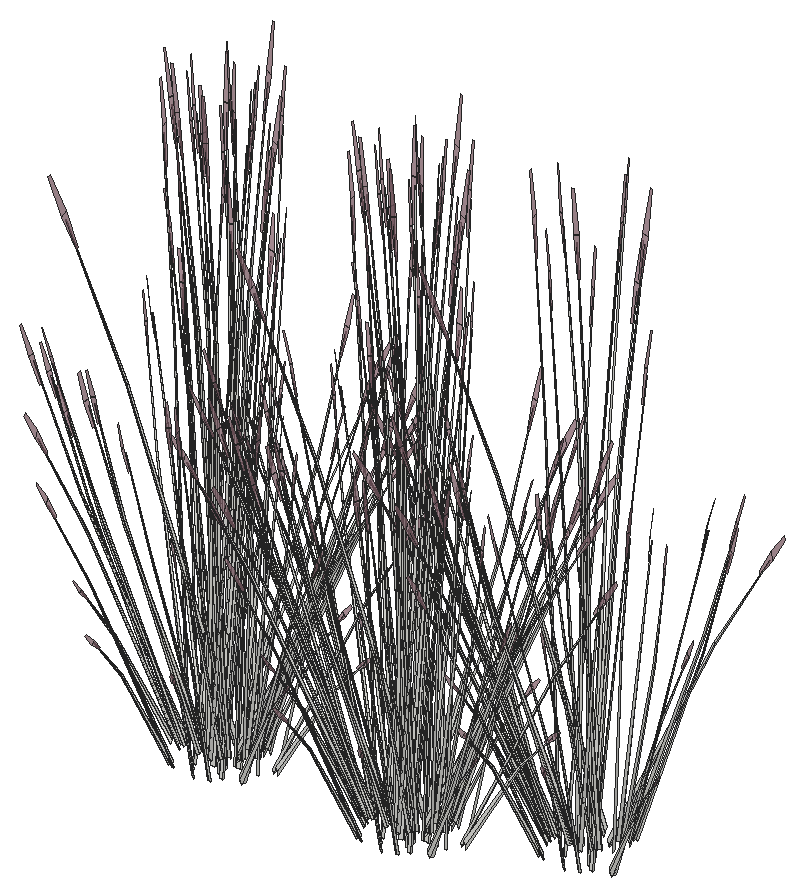
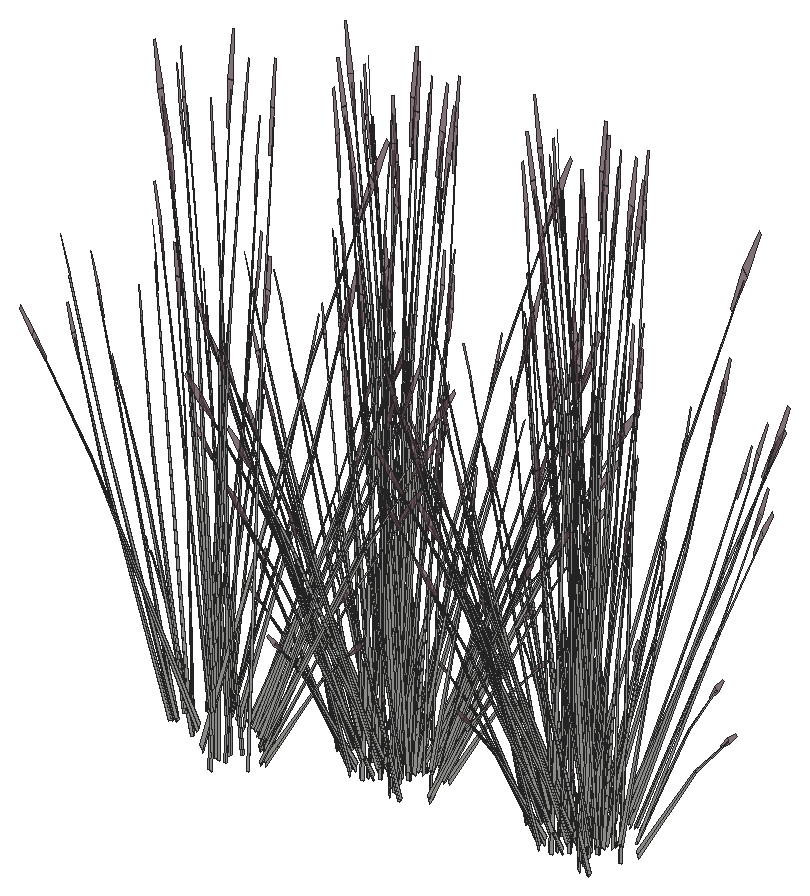
# SketchUp Ruby script. Lengths in inches.
U = 1.inch
M = Sketchup.active_model
def pt(a) = Geom::Point3d.new(a.map { |v| v * U })
def face(e, loops, mat)
  f = e.add_face(loops[0].map { |a| pt(a) })
  loops[1..].each { |l| e.add_face(l.map { |a| pt(a) }).erase! }
  f.material = f.back_material = mat if mat
  f
end
# faces: each face lists its corners as indices into pts; further lists are holes
def faces(e, pts, list, mat = nil) = list.each { |f| face(e, (f[0].is_a?(Array) ? f : [f]).map { |l| l.map { |i| pts[i] } }, mat) }
# xy, xz, yz: faces in a plane at the given z, y or x. An outline is a flat list of corners, or four numbers for a rectangle; further outlines are holes
def ring(l) = l.size == 4 ? [[l[0], l[1]], [l[2], l[1]], [l[2], l[3]], [l[0], l[3]]] : l.each_slice(2).to_a
def flat(e, list, mat, &to3) = list.each { |f| face(e, (f[0].is_a?(Array) ? f : [f]).map { |l| ring(l).map { |u, v| to3.(u, v) } }, mat) }
def xy(e, z, list, mat = nil) = flat(e, list, mat) { |x, y| [x, y, z] }
def xz(e, y, list, mat = nil) = flat(e, list, mat) { |x, z| [x, y, z] }
def yz(e, x, list, mat = nil) = flat(e, list, mat) { |y, z| [x, y, z] }
def lines(e, pts, list) = list.each { |a, b| e.add_line(pt(pts[a]), pt(pts[b])) }
# prism: a flat outline (further loops are holes) pulled along v
def prism(e, loops, v, mat = nil)
  f = face(e, loops, mat); d = Geom::Vector3d.new(v.map { |x| x * U })
  f.pushpull(f.normal.samedirection?(d) ? d.length : -d.length)
end
def box(e, o, s, mat = nil) = prism(e, [[o, [o[0] + s[0], o[1], o[2]], [o[0] + s[0], o[1] + s[1], o[2]], [o[0], o[1] + s[1], o[2]]]], [0, 0, s[2]], mat)
def at(x, y, z, deg = 0) = Geom::Transformation.translation(pt([x, y, z])) * Geom::Transformation.rotation(ORIGIN, Z_AXIS, deg.degrees)
def axes(o, x, y, z) = Geom::Transformation.new([*x, 0, *y, 0, *z, 0, *pt(o).to_a, 1])
def part(name) = M.definitions.add(name)
# library, detail: a bought-in or finely detailed component or shape, given as its bounding box
def library(name, o, s) = part(name).tap { |d| box(d.entities, o, s) }
def detail(e, o, s) = box(e.add_group.entities, o, s)
def put(e, d, t, mat = nil) = e.add_instance(d, t).tap { |i| i.material = mat if mat }
def group(e, t, mat = nil) = e.add_group.tap { |g| g.transformation = t; g.material = mat if mat }.entities
root = M.entities
M.materials.add("LightPink_Translucent").color = [144, 107, 117]
M.materials["LightPink_Translucent"].alpha = 0.75
c1 = part("blade")
p = [[2.15,0.21,22],[0,0.17,0],[0.09,0.45,0],[2.18,0.31,22],[2.29,0.31,22],[0.38,0.45,0],
  [2.48,0.24,33],[2.49,0.24,33],[2.48,0.22,33]]
faces(c1.entities,p,[[0,1,2,3],[4,5,2,3],[6,3,4,7],[8,0,3,6]])
c2 = part("seeds")
p = [[0.3,-0.1,1.38],[-0.01,-0.03,1.59],[-0.01,-0.03,0.03],[0.14,-0.07,-0.07],[0.29,-0.03,3],[0.15,0.01,3.11]]
faces(c2.entities,p,[[0,1,2,3],[1,0,4,5]],"LightPink_Translucent")
c3 = part("blade with seeds")
put(c3.entities,c1,at(0,0,0))
put(c3.entities,c2,axes([2.4,0.25,30.99],[1.5799,-0.05474,1.17369],[-0.12525,1.92788,0.29478],[-0.07173,-0.02425,1.56792]))
put(root,c3,axes([361.61,51.9,259.53],[-0.43232,-0.38257,-0.35414],[0.49364,-0.36215,0.4572],[-0.25081,-0.0551,0.87481]))
put(root,c3,axes([362.22,54.17,258.875],[0.18977,-0.18775,1.71376],[0.47917,0.50677,0.13857],[-0.32866,0.23079,0.73262]))
put(root,c3,axes([361.08,54.67,259.53],[-0.66138,0.08733,-0.35414],[-0.17464,-0.49921,0.4572],[-0.18953,0.13408,0.87481]))
put(root,c3,axes([360.57,52.82,257.77],[0.48508,-0.04372,1.1486],[-0.3077,0.38525,0.84392],[-0.23971,-0.05779,0.25299]))
put(root,c3,axes([362.08,54.64,258.875],[0.14147,-0.21002,1.71376],[0.59349,0.43464,0.13857],[-0.26773,0.27089,0.73262]))
put(root,c3,axes([361.625,54.72,259.68],[0.19519,0.55794,-0.51099],[-0.73919,0.0976,-0.3958],[-0.21183,0.14986,0.97773]))
put(root,c3,axes([363.39,51.43,259.98],[-0.64788,-0.29534,-0.71045],[0.46044,-0.51755,0.08574],[-0.23473,-0.17635,1.00501]))
put(root,c3,axes([363.09,51.44,259.68],[-0.74975,0.14525,-0.51099],[-0.13115,-0.55007,-0.3958],[-0.20138,-0.15763,0.97773]))
put(root,c3,axes([362.66,50.625,257.59],[-0.04601,0.19989,1.43002],[-0.67263,0.16733,-0.30754],[-0.15723,-0.25836,0.61141]))
put(root,c3,axes([362.88,51.14,258.875],[0.17368,0.19618,1.71376],[-0.80256,0.16516,0.13857],[-0.18139,-0.30799,0.73262]))
put(root,c3,axes([363.16,51.04,259.53],[-0.11735,-0.49217,-0.35414],[0.67083,-0.12996,0.4572],[-0.18018,-0.14104,0.87481]))
put(root,c3,axes([362.24,55.82,259.53],[-0.5141,0.32171,-0.35414],[-0.48666,-0.36734,0.4572],[-0.07405,0.18664,0.87481]))
put(root,c3,axes([364.9375,54.77,258.33],[0.65659,0.2464,1.51261],[-0.64324,0.53082,0.59816],[-0.28812,-0.31461,1.26806]))
put(root,c3,axes([362.43,50.3,257.77],[0.39634,0.21267,1.1486],[-0.57721,0.12784,0.84392],[-0.1235,-0.16344,0.25299]))
put(root,c3,axes([362.57,57.07,257.77],[-0.01966,-0.36332,1.1486],[0.49135,0.25914,0.84392],[-0.09663,0.17317,0.25299]))
put(root,c3,axes([363.27,55.54,257.48],[0.7111,0.30552,0.49651],[-0.42504,0.54784,0],[-0.16196,-0.06958,1.57504]))
put(root,c3,axes([364.29,54.59,257.62],[-0.14658,0.54532,0.1448],[-0.71613,-0.09466,-0.41347],[-0.13033,-0.05599,1.26744]))
put(root,c3,axes([361.87,53.63,257.48],[0,0.61104,0.49651],[-0.85008,0,0],[0,-0.13917,1.57504]))
put(root,c3,axes([362.75,55.67,260],[0.54391,0.41056,-0.5672],[-0.57458,0.35956,-0.43934],[-0.08276,0.2086,1.08528]))
put(root,c3,axes([365.96,53.59,257.84],[-0.02076,-0.57531,1.41272],[0.93937,0.14913,0.59816],[-0.22217,0.31481,1.3335]))
put(root,c3,axes([362.16,56.29,257.82],[0.69024,-0.1082,0.06507],[0.15868,0.43593,-0.86304],[-0.04376,0.22067,0.7736]))
put(root,c3,axes([364.75,51.1875,259.68],[-0.7469,-0.15318,-0.51099],[0.25601,-0.52518,-0.3958],[-0.06849,-0.21144,0.97773]))
put(root,c3,axes([364.05,54.07,257.36],[0.96033,0.12874,0.45755],[-0.19544,0.7271,0.17955],[-0.14034,-0.07021,1.58856]))
put(root,c3,axes([363.81,53.94,257.72],[-0.36864,0.55059,0.44739],[-0.76598,-0.26498,-0.21531],[0,-0.12692,1.43643]))
put(root,c3,axes([365.02,51.29,259.98],[-0.36264,-0.49684,-0.71045],[0.74649,-0.27689,0.08574],[-0.0848,-0.24006,1.00501]))
put(root,c3,axes([363.54,55.23,257.47],[0.81646,-0.16218,0.17642],[0.20161,0.60355,0.35086],[-0.07282,-0.08794,1.60407]))
put(root,c3,axes([365.97,55.27,257.47],[0.21949,-0.60727,0.17642],[0.8032,0.17185,0.35086],[-0.13875,0.00296,1.60407]))
put(root,c3,axes([365.6,54.46,257.62],[0.56134,0.36712,0.1448],[-0.46823,0.41419,-0.41347],[-0.13033,0.05599,1.26744]))
put(root,c3,axes([365.58,54.19,257.72],[0.82508,-0.03772,0.44739],[0.07462,0.62614,-0.21531],[-0.14771,0.06346,1.43643]))
put(root,c3,axes([366.19,55.59,257.48],[0.7111,-0.30552,0.49651],[0.42504,0.54784,0],[-0.16196,0.06958,1.57504]))
put(root,c3,axes([365.09,50.87,259.53],[0.22906,-0.4699,-0.35414],[0.66828,0.13705,0.4572],[-0.06128,-0.18919,0.87481]))
put(root,c3,axes([363.97,53.4,257.36],[0.33034,0.68327,0.45755],[-0.94388,0.2376,0.17955],[0.01154,-0.12555,1.58856]))
put(root,c3,axes([367.22,53.72,257.47],[-0.59697,-0.44509,0.17642],[0.60159,-0.4317,0.35086],[-0.06593,0.0909,1.60407]))
put(root,c3,axes([364.28,53.59,257.43],[0.8561,0.29616,0.24065],[-0.41201,0.61537,0.50002],[0,-0.14185,1.60543]))
put(root,c3,axes([364,53.18,257.72],[-0.82508,0.03772,0.44739],[-0.07462,-0.62614,-0.21531],[0.14771,-0.06346,1.43643]))
put(root,c3,axes([363.62,52.1,257.47],[-0.21949,0.60727,0.17642],[-0.8032,-0.17185,0.35086],[0.13875,-0.00296,1.60407]))
put(root,c3,axes([366.05,52.14,257.47],[-0.81646,0.16218,0.17642],[-0.20161,-0.60355,0.35086],[0.07282,0.08794,1.60407]))
put(root,c3,axes([365.21,49.875,257.77],[0.09747,0.35631,1.1486],[-0.54071,-0.19735,0.84392],[0.05818,-0.18244,0.25299]))
put(root,c3,axes([364.71,53.02,257.36],[-0.62999,0.55453,0.45755],[-0.74845,-0.4895,0.17955],[0.15188,-0.05534,1.58856]))
put(root,c3,axes([365.78,53.43,257.72],[0.36864,-0.55059,0.44739],[0.76598,0.26498,-0.21531],[0,0.12692,1.43643]))
put(root,c3,axes([364.37,56.07,259.68],[0.7469,0.15318,-0.51099],[-0.25601,0.52518,-0.3958],[0.06849,0.21144,0.97773]))
put(root,c3,axes([365.53,53.3,257.38],[-0.96033,-0.12874,0.49198],[0.19544,-0.7271,0.19306],[0.14034,0.07021,1.70813]))
put(root,c3,axes([364.99,52.92,257.72],[-0.45644,-0.51287,0.44739],[0.69137,-0.36116,-0.21531],[0.14771,0.06346,1.43643]))
put(root,c3,axes([366.1,53.55,257.62],[0.70791,-0.1782,0.1448],[0.24791,0.50885,-0.41347],[0,0.11199,1.26744]))
put(root,c3,axes([366.36,51.59,259.68],[-0.54391,-0.41056,-0.51099],[0.57458,-0.35956,-0.3958],[0.08276,-0.2086,0.97773]))
put(root,c3,axes([366.01,50.86,257.59],[-0.21597,0.12368,1.43002],[-0.64681,-0.21647,-0.30754],[0.1199,-0.26922,0.61141]))
put(root,c3,axes([367.71,53.74,257.48],[0,-0.61104,0.49651],[0.85008,0,0],[0,0.13917,1.57504]))
put(root,c3,axes([364.79,54.98,258.875],[-0.17368,-0.19618,1.71376],[0.80256,-0.16516,0.13857],[0.18139,0.30799,0.73262]))
put(root,c3,axes([365.29,52.78,257.62],[0.14658,-0.54532,0.1448],[0.71613,0.09466,-0.41347],[0.13033,0.05599,1.26744]))
put(root,c3,axes([366.3125,51.83,257.48],[-0.7111,-0.30552,0.49651],[0.42504,-0.54784,0],[0.16196,0.06958,1.57504]))
put(root,c3,axes([366.53,51.77,259.98],[0.01977,-0.56521,-0.71045],[0.83252,0.03796,0.08574],[0.08786,-0.23945,1.00501]))
put(root,c3,axes([366.875,51.43,259.53],[0.5141,-0.32171,-0.35414],[0.48666,0.36734,0.4572],[0.07405,-0.18664,0.87481]))
put(root,c3,axes([367,55.57,257.77],[-0.4278,-0.1757,1.1486],[0.5524,-0.17852,0.84392],[0.14899,0.15122,0.25299]))
put(root,c3,axes([365.48,55.38,257.59],[0.01341,-0.20255,1.43002],[0.64074,-0.22625,-0.30754],[0.1978,0.24243,0.61141]))
put(root,c3,axes([367.07,56.37,257.67],[-0.48723,-0.01916,1.0506],[0.32177,-0.40701,0.58006],[0.19248,0.1446,0.8241]))
put(root,c3,axes([365.6,51.49,258.875],[-0.14147,0.21002,1.71376],[-0.59349,-0.43464,0.13857],[0.26773,-0.27089,0.73262]))
put(root,c3,axes([366.03,55.8125,259.68],[0.74975,-0.14525,-0.51099],[0.13115,0.55007,-0.3958],[0.20138,0.15763,0.97773]))
put(root,c3,axes([378.76,52.72,258.875],[0.31515,-0.01384,1.71376],[-0.20907,0.5998,0.13857],[-0.44912,-0.0371,0.73262]))
put(root,c3,axes([367.49,52.53,259.68],[-0.19519,-0.55794,-0.51099],[0.73919,-0.0976,-0.3958],[0.21183,-0.14986,0.97773]))
put(root,c3,axes([368.79,55.41,258.93],[-0.14542,-0.51365,-0.03492],[0.68734,-0.11809,-0.15832],[0.14353,0.03256,0.52218]))
put(root,c3,axes([368.4,51.42,257.77],[-0.25308,0.31105,1.1486],[-0.21753,-0.4179,0.84392],[0.20902,-0.10472,0.25299]))
put(root,c3,axes([378.89,53.77,258.875],[0.26363,-0.12925,1.71376],[0.22195,0.59723,0.13857],[-0.41388,0.13498,0.73262]))
put(root,c3,axes([378.07,54.79,257.59],[0.26405,0.05016,1.43002],[0.17019,0.51235,-0.30754],[-0.35868,0.0959,0.61141]))
put(root,c3,axes([365.95,54.37,258.875],[-0.28223,-0.10528,1.71376],[0.58406,-0.44165,0.13857],[0.36402,0.19924,0.73262]))
put(root,c3,axes([380.41,53.15,258.34],[0.21597,-0.08839,1.77064],[0.07448,0.61717,0.13857],[-0.4678,0.08189,0.63284]))
put(root,c3,axes([368.04,52.59,259.53],[0.66138,-0.08733,-0.35414],[0.17464,0.49921,0.4572],[0.18953,-0.13408,0.87481]))
put(root,c3,axes([367.51,52.76,259.98],[0.39688,-0.48213,-0.71045],[0.69548,0.34264,0.08574],[0.23697,-0.17468,1.00501]))
put(root,c3,axes([367.51,55.35,259.53],[0.43232,0.38257,-0.35414],[-0.49364,0.36215,0.4572],[0.25081,0.0551,0.87481]))
put(root,c3,axes([379.7,52.16,259.98],[-0.75952,-0.01471,-0.71045],[0.05101,-0.61953,0.08574],[-0.32177,-0.06538,1.00501]))
put(root,c3,axes([379.09,52.31,257.59],[0.14835,0.17012,1.43002],[-0.34183,0.46242,-0.30754],[-0.351,-0.11053,0.61141]))
put(root,c3,axes([378.48,53.23,259.53],[-0.63144,-0.17046,-0.35414],[0.18417,-0.49731,0.4572],[-0.25423,0.0456,0.87481]))
put(root,c3,axes([379.36,51.75,258.875],[0.28223,0.10528,1.71376],[-0.58406,0.44165,0.13857],[-0.36402,-0.19924,0.73262]))
put(root,c3,axes([378.92,53.49,259.68],[-0.20584,0.55581,-0.51099],[-0.70573,-0.19051,-0.3958],[-0.28414,0.05097,0.97773]))
put(root,c3,axes([367.84,53.77,259.68],[0.20584,-0.55581,-0.51099],[0.70573,0.19051,-0.3958],[0.28414,-0.05097,0.97773]))
put(root,c3,axes([379.45,52.28,259.68],[-0.55171,0.40476,-0.51099],[-0.48318,-0.42758,-0.3958],[-0.28031,-0.06159,0.97773]))
put(root,c3,axes([369.61,54.125,257.77],[-0.46945,0.10088,1.1486],[0.22097,-0.4169,0.84392],[0.24904,0.02853,0.25299]))
put(root,c3,axes([368.09,52.3125,257.59],[-0.27143,-0.0181,1.43002],[-0.27808,-0.48551,-0.30754],[0.33346,-0.13735,0.61141]))
put(root,c3,axes([368.27,54.02,259.53],[0.63144,0.17046,-0.35414],[-0.18417,0.49731,0.4572],[0.25423,-0.0456,0.87481]))
put(root,c3,axes([377.52,55.86,257.77],[0.31665,-0.27694,1.1486],[0.12495,0.43841,0.84392],[-0.22883,0.0785,0.25299]))
put(root,c3,axes([367.05,55.1,259.98],[0.75952,0.01471,-0.71045],[-0.05101,0.61953,0.08574],[0.32177,0.06538,1.00501]))
put(root,c3,axes([379.25,51.9,259.53],[-0.43232,-0.38257,-0.35414],[0.49364,-0.36215,0.4572],[-0.25081,-0.0551,0.87481]))
put(root,c3,axes([366.55,53.41,258.875],[-0.31515,0.01384,1.71376],[0.20907,-0.5998,0.13857],[0.44912,0.0371,0.73262]))
put(root,c3,axes([379.86,54.17,258.875],[0.18977,-0.18775,1.71376],[0.47917,0.50677,0.13857],[-0.32866,0.23079,0.73262]))
put(root,c3,axes([378.71,54.67,259.53],[-0.66138,0.08733,-0.35414],[-0.17464,-0.49921,0.4572],[-0.18953,0.13408,0.87481]))
put(root,c3,axes([378.21,52.82,257.77],[0.48508,-0.04372,1.1486],[-0.3077,0.38525,0.84392],[-0.23971,-0.05779,0.25299]))
put(root,c3,axes([367.7,53.97,259.98],[0.66765,-0.26986,-0.71045],[0.37208,0.55551,0.08574],[0.32259,-0.0631,1.00501]))
put(root,c3,axes([379.71,54.64,258.875],[0.14147,-0.21002,1.71376],[0.59349,0.43464,0.13857],[-0.26773,0.27089,0.73262]))
put(root,c3,axes([368.73,54.79,257.59],[-0.18299,-0.15028,1.43002],[0.23809,-0.49714,-0.30754],[0.37023,0.06735,0.61141]))
put(root,c3,axes([379.26,54.72,259.68],[0.19519,0.55794,-0.51099],[-0.73919,0.0976,-0.3958],[-0.21183,0.14986,0.97773]))
put(root,c3,axes([381.02,51.43,259.98],[-0.64788,-0.29534,-0.71045],[0.46044,-0.51755,0.08574],[-0.23473,-0.17635,1.00501]))
put(root,c3,axes([380.72,51.44,259.68],[-0.74975,0.14525,-0.51099],[-0.13115,-0.55007,-0.3958],[-0.20138,-0.15763,0.97773]))
put(root,c3,axes([380.3,50.625,257.59],[-0.04601,0.19989,1.43002],[-0.67263,0.16733,-0.30754],[-0.15723,-0.25836,0.61141]))
put(root,c3,axes([380.52,51.14,258.875],[0.17368,0.19618,1.71376],[-0.80256,0.16516,0.13857],[-0.18139,-0.30799,0.73262]))
put(root,c3,axes([380.8,51.04,259.53],[-0.11735,-0.49217,-0.35414],[0.67083,-0.12996,0.4572],[-0.18018,-0.14104,0.87481]))
put(root,c3,axes([379.88,55.82,259.53],[-0.5141,0.32171,-0.35414],[-0.48666,-0.36734,0.4572],[-0.07405,0.18664,0.87481]))
put(root,c3,axes([382.57,54.77,258.33],[0.65659,0.2464,1.51261],[-0.64324,0.53082,0.59816],[-0.28812,-0.31461,1.26806]))
put(root,c3,axes([380.07,50.3,257.77],[0.39634,0.21267,1.1486],[-0.57721,0.12784,0.84392],[-0.1235,-0.16344,0.25299]))
put(root,c3,axes([380.21,57.07,257.77],[-0.01966,-0.36332,1.1486],[0.49135,0.25914,0.84392],[-0.09663,0.17317,0.25299]))
put(root,c3,axes([380.91,55.54,257.48],[0.7111,0.30552,0.49651],[-0.42504,0.54784,0],[-0.16196,-0.06958,1.57504]))
put(root,c3,axes([381.93,54.59,257.62],[-0.14658,0.54532,0.1448],[-0.71613,-0.09466,-0.41347],[-0.13033,-0.05599,1.26744]))
put(root,c3,axes([379.51,53.63,257.48],[0,0.61104,0.49651],[-0.85008,0,0],[0,-0.13917,1.57504]))
put(root,c3,axes([380.39,55.67,260],[0.54391,0.41056,-0.5672],[-0.57458,0.35956,-0.43934],[-0.08276,0.2086,1.08528]))
put(root,c3,axes([383.59,53.59,257.84],[-0.02076,-0.57531,1.41272],[0.93937,0.14913,0.59816],[-0.22217,0.31481,1.3335]))
put(root,c3,axes([379.8,56.29,257.82],[0.69024,-0.1082,0.06507],[0.15868,0.43593,-0.86304],[-0.04376,0.22067,0.7736]))
put(root,c3,axes([382.39,51.1875,259.68],[-0.7469,-0.15318,-0.51099],[0.25601,-0.52518,-0.3958],[-0.06849,-0.21144,0.97773]))
put(root,c3,axes([381.69,54.07,257.36],[0.96033,0.12874,0.45755],[-0.19544,0.7271,0.17955],[-0.14034,-0.07021,1.58856]))
put(root,c3,axes([381.44,53.94,257.72],[-0.36864,0.55059,0.44739],[-0.76598,-0.26498,-0.21531],[0,-0.12692,1.43643]))
put(root,c3,axes([382.66,51.29,259.98],[-0.36264,-0.49684,-0.71045],[0.74649,-0.27689,0.08574],[-0.0848,-0.24006,1.00501]))
put(root,c3,axes([381.17,55.23,257.47],[0.81646,-0.16218,0.17642],[0.20161,0.60355,0.35086],[-0.07282,-0.08794,1.60407]))
put(root,c3,axes([383.6,55.27,257.47],[0.21949,-0.60727,0.17642],[0.8032,0.17185,0.35086],[-0.13875,0.00296,1.60407]))
put(root,c3,axes([383.23,54.46,257.62],[0.56134,0.36712,0.1448],[-0.46823,0.41419,-0.41347],[-0.13033,0.05599,1.26744]))
put(root,c3,axes([383.22,54.19,257.72],[0.82508,-0.03772,0.44739],[0.07462,0.62614,-0.21531],[-0.14771,0.06346,1.43643]))
put(root,c3,axes([383.83,55.59,257.48],[0.7111,-0.30552,0.49651],[0.42504,0.54784,0],[-0.16196,0.06958,1.57504]))
put(root,c3,axes([382.73,50.87,259.53],[0.22906,-0.4699,-0.35414],[0.66828,0.13705,0.4572],[-0.06128,-0.18919,0.87481]))
put(root,c3,axes([381.61,53.4,257.36],[0.33034,0.68327,0.45755],[-0.94388,0.2376,0.17955],[0.01154,-0.12555,1.58856]))
put(root,c3,axes([384.86,53.72,257.47],[-0.59697,-0.44509,0.17642],[0.60159,-0.4317,0.35086],[-0.06593,0.0909,1.60407]))
put(root,c3,axes([381.91,53.59,257.43],[0.8561,0.29616,0.24065],[-0.41201,0.61537,0.50002],[0,-0.14185,1.60543]))
put(root,c3,axes([381.64,53.18,257.72],[-0.82508,0.03772,0.44739],[-0.07462,-0.62614,-0.21531],[0.14771,-0.06346,1.43643]))
put(root,c3,axes([390.89,58.94,258.875],[0.31515,-0.01384,1.71376],[-0.20907,0.5998,0.13857],[-0.44912,-0.0371,0.73262]))
put(root,c3,axes([381.25,52.1,257.47],[-0.21949,0.60727,0.17642],[-0.8032,-0.17185,0.35086],[0.13875,-0.00296,1.60407]))
put(root,c3,axes([383.68,52.14,257.47],[-0.81646,0.16218,0.17642],[-0.20161,-0.60355,0.35086],[0.07282,0.08794,1.60407]))
put(root,c3,axes([382.85,49.875,257.77],[0.09747,0.35631,1.1486],[-0.54071,-0.19735,0.84392],[0.05818,-0.18244,0.25299]))
put(root,c3,axes([382.35,53.02,257.36],[-0.62999,0.55453,0.45755],[-0.74845,-0.4895,0.17955],[0.15188,-0.05534,1.58856]))
put(root,c3,axes([383.41,53.43,257.72],[0.36864,-0.55059,0.44739],[0.76598,0.26498,-0.21531],[0,0.12692,1.43643]))
put(root,c3,axes([382,56.07,259.68],[0.7469,0.15318,-0.51099],[-0.25601,0.52518,-0.3958],[0.06849,0.21144,0.97773]))
put(root,c3,axes([383.17,53.3,257.38],[-0.96033,-0.12874,0.49198],[0.19544,-0.7271,0.19306],[0.14034,0.07021,1.70813]))
put(root,c3,axes([382.62,52.92,257.72],[-0.45644,-0.51287,0.44739],[0.69137,-0.36116,-0.21531],[0.14771,0.06346,1.43643]))
put(root,c3,axes([383.73,53.55,257.62],[0.70791,-0.1782,0.1448],[0.24791,0.50885,-0.41347],[0,0.11199,1.26744]))
put(root,c3,axes([384,51.59,259.68],[-0.54391,-0.41056,-0.51099],[0.57458,-0.35956,-0.3958],[0.08276,-0.2086,0.97773]))
put(root,c3,axes([391.83,58.39,259.98],[-0.75952,-0.01471,-0.71045],[0.05101,-0.61953,0.08574],[-0.32177,-0.06538,1.00501]))
put(root,c3,axes([391.22,58.54,257.59],[0.14835,0.17012,1.43002],[-0.34183,0.46242,-0.30754],[-0.351,-0.11053,0.61141]))
put(root,c3,axes([390.61,59.46,259.53],[-0.63144,-0.17046,-0.35414],[0.18417,-0.49731,0.4572],[-0.25423,0.0456,0.87481]))
put(root,c3,axes([391.49,57.98,258.875],[0.28223,0.10528,1.71376],[-0.58406,0.44165,0.13857],[-0.36402,-0.19924,0.73262]))
put(root,c3,axes([383.64,50.86,257.59],[-0.21597,0.12368,1.43002],[-0.64681,-0.21647,-0.30754],[0.1199,-0.26922,0.61141]))
put(root,c3,axes([385.35,53.74,257.48],[0,-0.61104,0.49651],[0.85008,0,0],[0,0.13917,1.57504]))
put(root,c3,axes([391.58,58.51,259.68],[-0.55171,0.40476,-0.51099],[-0.48318,-0.42758,-0.3958],[-0.28031,-0.06159,0.97773]))
put(root,c3,axes([382.43,54.98,258.875],[-0.17368,-0.19618,1.71376],[0.80256,-0.16516,0.13857],[0.18139,0.30799,0.73262]))
put(root,c3,axes([382.93,52.78,257.62],[0.14658,-0.54532,0.1448],[0.71613,0.09466,-0.41347],[0.13033,0.05599,1.26744]))
put(root,c3,axes([383.95,51.83,257.48],[-0.7111,-0.30552,0.49651],[0.42504,-0.54784,0],[0.16196,0.06958,1.57504]))
put(root,c3,axes([384.17,51.77,259.98],[0.01977,-0.56521,-0.71045],[0.83252,0.03796,0.08574],[0.08786,-0.23945,1.00501]))
put(root,c3,axes([391.38,58.13,259.53],[-0.43232,-0.38257,-0.35414],[0.49364,-0.36215,0.4572],[-0.25081,-0.0551,0.87481]))
put(root,c3,axes([390.34,59.05,257.77],[0.48508,-0.04372,1.1486],[-0.3077,0.38525,0.84392],[-0.23971,-0.05779,0.25299]))
put(root,c3,axes([384.51,51.43,259.53],[0.5141,-0.32171,-0.35414],[0.48666,0.36734,0.4572],[0.07405,-0.18664,0.87481]))
put(root,c3,axes([384.63,55.57,257.77],[-0.4278,-0.1757,1.1486],[0.5524,-0.17852,0.84392],[0.14899,0.15122,0.25299]))
put(root,c3,axes([383.11,55.38,257.59],[0.01341,-0.20255,1.43002],[0.64074,-0.22625,-0.30754],[0.1978,0.24243,0.61141]))
put(root,c3,axes([384.7,56.37,257.67],[-0.48723,-0.01916,1.0506],[0.32177,-0.40701,0.58006],[0.19248,0.1446,0.8241]))
put(root,c3,axes([383.23,51.49,258.875],[-0.14147,0.21002,1.71376],[-0.59349,-0.43464,0.13857],[0.26773,-0.27089,0.73262]))
put(root,c3,axes([393.16,57.66,259.98],[-0.64788,-0.29534,-0.71045],[0.46044,-0.51755,0.08574],[-0.23473,-0.17635,1.00501]))
put(root,c3,axes([392.85,57.67,259.68],[-0.74975,0.14525,-0.51099],[-0.13115,-0.55007,-0.3958],[-0.20138,-0.15763,0.97773]))
put(root,c3,axes([383.67,55.8125,259.68],[0.74975,-0.14525,-0.51099],[0.13115,0.55007,-0.3958],[0.20138,0.15763,0.97773]))
put(root,c3,axes([385.13,52.53,259.68],[-0.19519,-0.55794,-0.51099],[0.73919,-0.0976,-0.3958],[0.21183,-0.14986,0.97773]))
put(root,c3,axes([386.43,55.41,258.93],[-0.14542,-0.51365,-0.03492],[0.68734,-0.11809,-0.15832],[0.14353,0.03256,0.52218]))
put(root,c3,axes([392.43,56.85,257.59],[-0.04601,0.19989,1.43002],[-0.67263,0.16733,-0.30754],[-0.15723,-0.25836,0.61141]))
put(root,c3,axes([386.04,51.42,257.77],[-0.25308,0.31105,1.1486],[-0.21753,-0.4179,0.84392],[0.20902,-0.10472,0.25299]))
put(root,c3,axes([392.65,57.37,258.875],[0.17368,0.19618,1.71376],[-0.80256,0.16516,0.13857],[-0.18139,-0.30799,0.73262]))
put(root,c3,axes([392.93,57.27,259.53],[-0.11735,-0.49217,-0.35414],[0.67083,-0.12996,0.4572],[-0.18018,-0.14104,0.87481]))
put(root,c3,axes([383.59,54.37,258.875],[-0.28223,-0.10528,1.71376],[0.58406,-0.44165,0.13857],[0.36402,0.19924,0.73262]))
put(root,c3,axes([385.67,52.59,259.53],[0.66138,-0.08733,-0.35414],[0.17464,0.49921,0.4572],[0.18953,-0.13408,0.87481]))
put(root,c3,axes([385.15,52.76,259.98],[0.39688,-0.48213,-0.71045],[0.69548,0.34264,0.08574],[0.23697,-0.17468,1.00501]))
put(root,c3,axes([385.14,55.35,259.53],[0.43232,0.38257,-0.35414],[-0.49364,0.36215,0.4572],[0.25081,0.0551,0.87481]))
put(root,c3,axes([394.71,61,258.33],[0.65659,0.2464,1.51261],[-0.64324,0.53082,0.59816],[-0.28812,-0.31461,1.26806]))
put(root,c3,axes([392.2,56.53,257.77],[0.39634,0.21267,1.1486],[-0.57721,0.12784,0.84392],[-0.1235,-0.16344,0.25299]))
put(root,c3,axes([385.47,53.77,259.68],[0.20584,-0.55581,-0.51099],[0.70573,0.19051,-0.3958],[0.28414,-0.05097,0.97773]))
put(root,c3,axes([387.24,54.125,257.77],[-0.46945,0.10088,1.1486],[0.22097,-0.4169,0.84392],[0.24904,0.02853,0.25299]))
put(root,c3,axes([385.72,52.3125,257.59],[-0.27143,-0.0181,1.43002],[-0.27808,-0.48551,-0.30754],[0.33346,-0.13735,0.61141]))
put(root,c3,axes([385.91,54.02,259.53],[0.63144,0.17046,-0.35414],[-0.18417,0.49731,0.4572],[0.25423,-0.0456,0.87481]))
put(root,c3,axes([391.64,59.86,257.48],[0,0.61104,0.49651],[-0.85008,0,0],[0,-0.13917,1.57504]))
put(root,c3,axes([384.69,55.1,259.98],[0.75952,0.01471,-0.71045],[-0.05101,0.61953,0.08574],[0.32177,0.06538,1.00501]))
put(root,c3,axes([384.18,53.41,258.875],[-0.31515,0.01384,1.71376],[0.20907,-0.5998,0.13857],[0.44912,0.0371,0.73262]))
put(root,c3,axes([385.34,53.97,259.98],[0.66765,-0.26986,-0.71045],[0.37208,0.55551,0.08574],[0.32259,-0.0631,1.00501]))
put(root,c3,axes([394.52,57.42,259.68],[-0.7469,-0.15318,-0.51099],[0.25601,-0.52518,-0.3958],[-0.06849,-0.21144,0.97773]))
put(root,c3,axes([386.36,54.79,257.59],[-0.18299,-0.15028,1.43002],[0.23809,-0.49714,-0.30754],[0.37023,0.06735,0.61141]))
put(root,c3,axes([393.57,60.17,257.72],[-0.36864,0.55059,0.44739],[-0.76598,-0.26498,-0.21531],[0,-0.12692,1.43643]))
put(root,c3,axes([394.79,57.52,259.98],[-0.36264,-0.49684,-0.71045],[0.74649,-0.27689,0.08574],[-0.0848,-0.24006,1.00501]))
put(root,c3,axes([393.31,61.46,257.47],[0.81646,-0.16218,0.17642],[0.20161,0.60355,0.35086],[-0.07282,-0.08794,1.60407]))
put(root,c3,axes([394.86,57.09,259.53],[0.22906,-0.4699,-0.35414],[0.66828,0.13705,0.4572],[-0.06128,-0.18919,0.87481]))
put(root,c3,axes([394.04,59.82,257.43],[0.8561,0.29616,0.24065],[-0.41201,0.61537,0.50002],[0,-0.14185,1.60543]))
put(root,c3,axes([393.77,59.4,257.72],[-0.82508,0.03772,0.44739],[-0.07462,-0.62614,-0.21531],[0.14771,-0.06346,1.43643]))
put(root,c3,axes([393.38,58.33,257.47],[-0.21949,0.60727,0.17642],[-0.8032,-0.17185,0.35086],[0.13875,-0.00296,1.60407]))
put(root,c3,axes([395.8125,58.36,257.47],[-0.81646,0.16218,0.17642],[-0.20161,-0.60355,0.35086],[0.07282,0.08794,1.60407]))
put(root,c3,axes([394.98,56.1,257.77],[0.09747,0.35631,1.1486],[-0.54071,-0.19735,0.84392],[0.05818,-0.18244,0.25299]))
put(root,c3,axes([394.75,59.15,257.72],[-0.45644,-0.51287,0.44739],[0.69137,-0.36116,-0.21531],[0.14771,0.06346,1.43643]))
put(root,c3,axes([396.13,57.8125,259.68],[-0.54391,-0.41056,-0.51099],[0.57458,-0.35956,-0.3958],[0.08276,-0.2086,0.97773]))
put(root,c3,axes([395.77,57.08,257.59],[-0.21597,0.12368,1.43002],[-0.64681,-0.21647,-0.30754],[0.1199,-0.26922,0.61141]))
put(root,c3,axes([395.06,59,257.62],[0.14658,-0.54532,0.1448],[0.71613,0.09466,-0.41347],[0.13033,0.05599,1.26744]))
put(root,c3,axes([396.08,58.05,257.48],[-0.7111,-0.30552,0.49651],[0.42504,-0.54784,0],[0.16196,0.06958,1.57504]))
put(root,c3,axes([396.3,58,259.98],[0.01977,-0.56521,-0.71045],[0.83252,0.03796,0.08574],[0.08786,-0.23945,1.00501]))
put(root,c3,axes([396.64,57.66,259.53],[0.5141,-0.32171,-0.35414],[0.48666,0.36734,0.4572],[0.07405,-0.18664,0.87481]))
put(root,c3,axes([395.36,57.71,258.875],[-0.14147,0.21002,1.71376],[-0.59349,-0.43464,0.13857],[0.26773,-0.27089,0.73262]))
put(root,c3,axes([397.26,58.76,259.68],[-0.19519,-0.55794,-0.51099],[0.73919,-0.0976,-0.3958],[0.21183,-0.14986,0.97773]))
put(root,c3,axes([398.17,57.65,257.77],[-0.25308,0.31105,1.1486],[-0.21753,-0.4179,0.84392],[0.20902,-0.10472,0.25299]))
put(root,c3,axes([397.81,58.82,259.53],[0.66138,-0.08733,-0.35414],[0.17464,0.49921,0.4572],[0.18953,-0.13408,0.87481]))
put(root,c3,axes([397.28,58.98,259.98],[0.39688,-0.48213,-0.71045],[0.69548,0.34264,0.08574],[0.23697,-0.17468,1.00501]))
put(root,c3,axes([397.6,60,259.68],[0.20584,-0.55581,-0.51099],[0.70573,0.19051,-0.3958],[0.28414,-0.05097,0.97773]))
put(root,c3,axes([397.85,58.54,257.59],[-0.27143,-0.0181,1.43002],[-0.27808,-0.48551,-0.30754],[0.33346,-0.13735,0.61141]))
put(root,c3,axes([398.04,60.25,259.53],[0.63144,0.17046,-0.35414],[-0.18417,0.49731,0.4572],[0.25423,-0.0456,0.87481]))
put(root,c3,axes([396.32,59.64,258.875],[-0.31515,0.01384,1.71376],[0.20907,-0.5998,0.13857],[0.44912,0.0371,0.73262]))
put(root,c3,axes([397.47,60.2,259.98],[0.66765,-0.26986,-0.71045],[0.37208,0.55551,0.08574],[0.32259,-0.0631,1.00501]))
